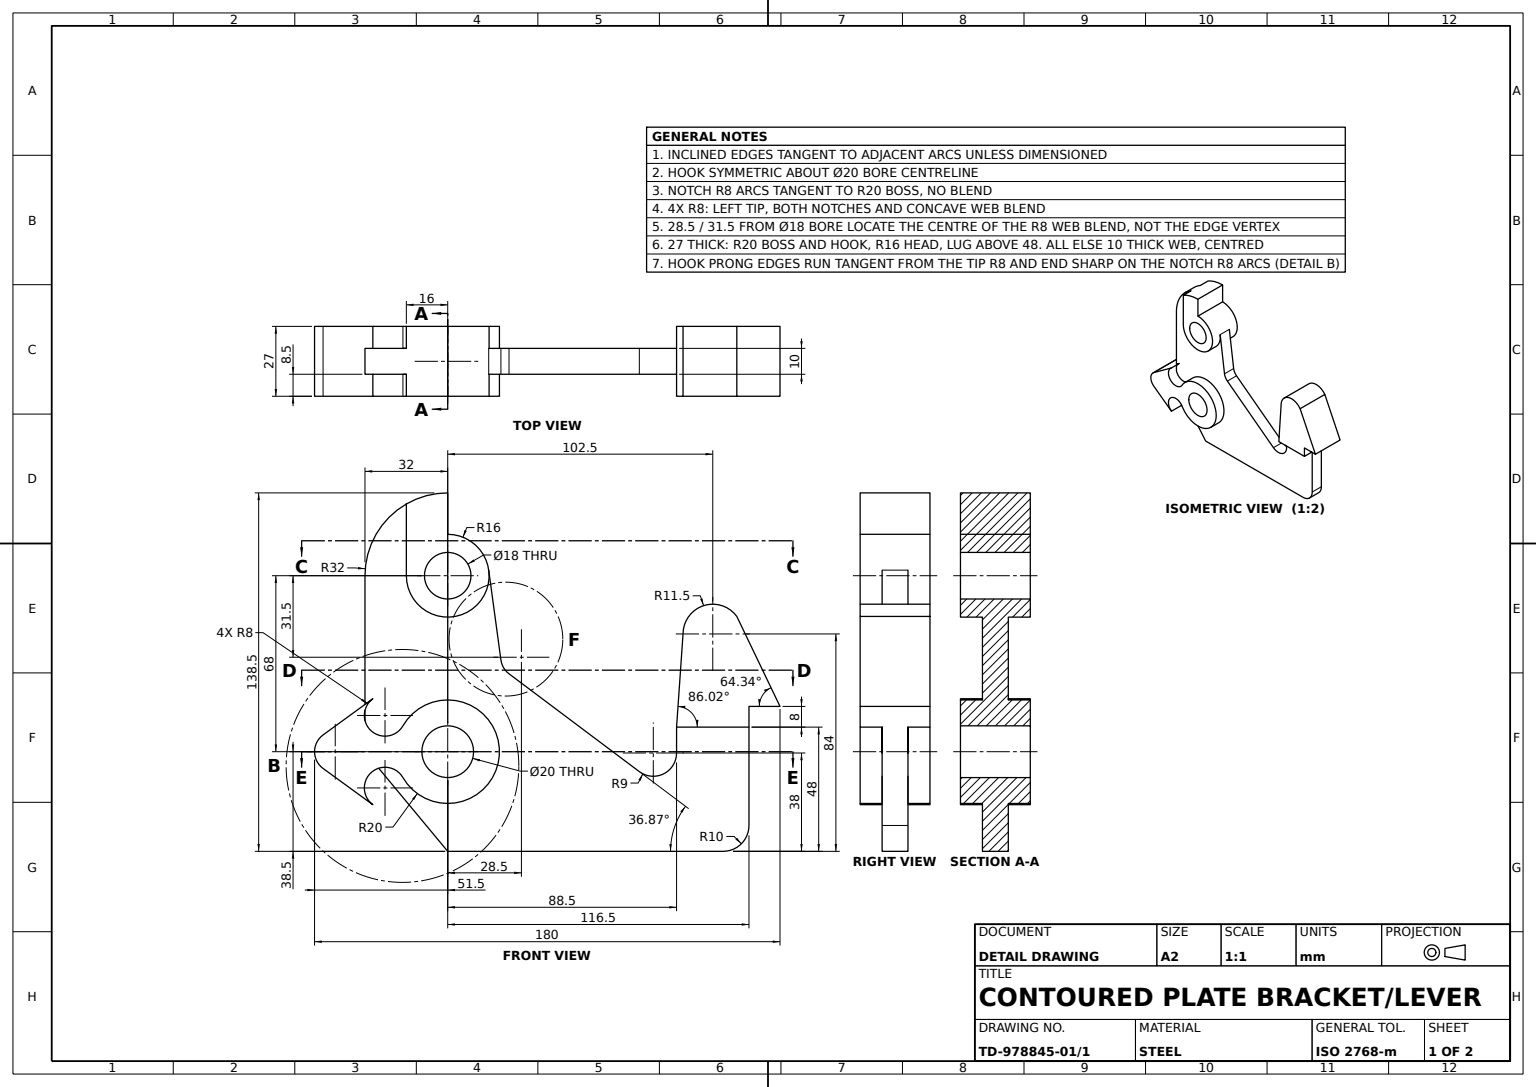
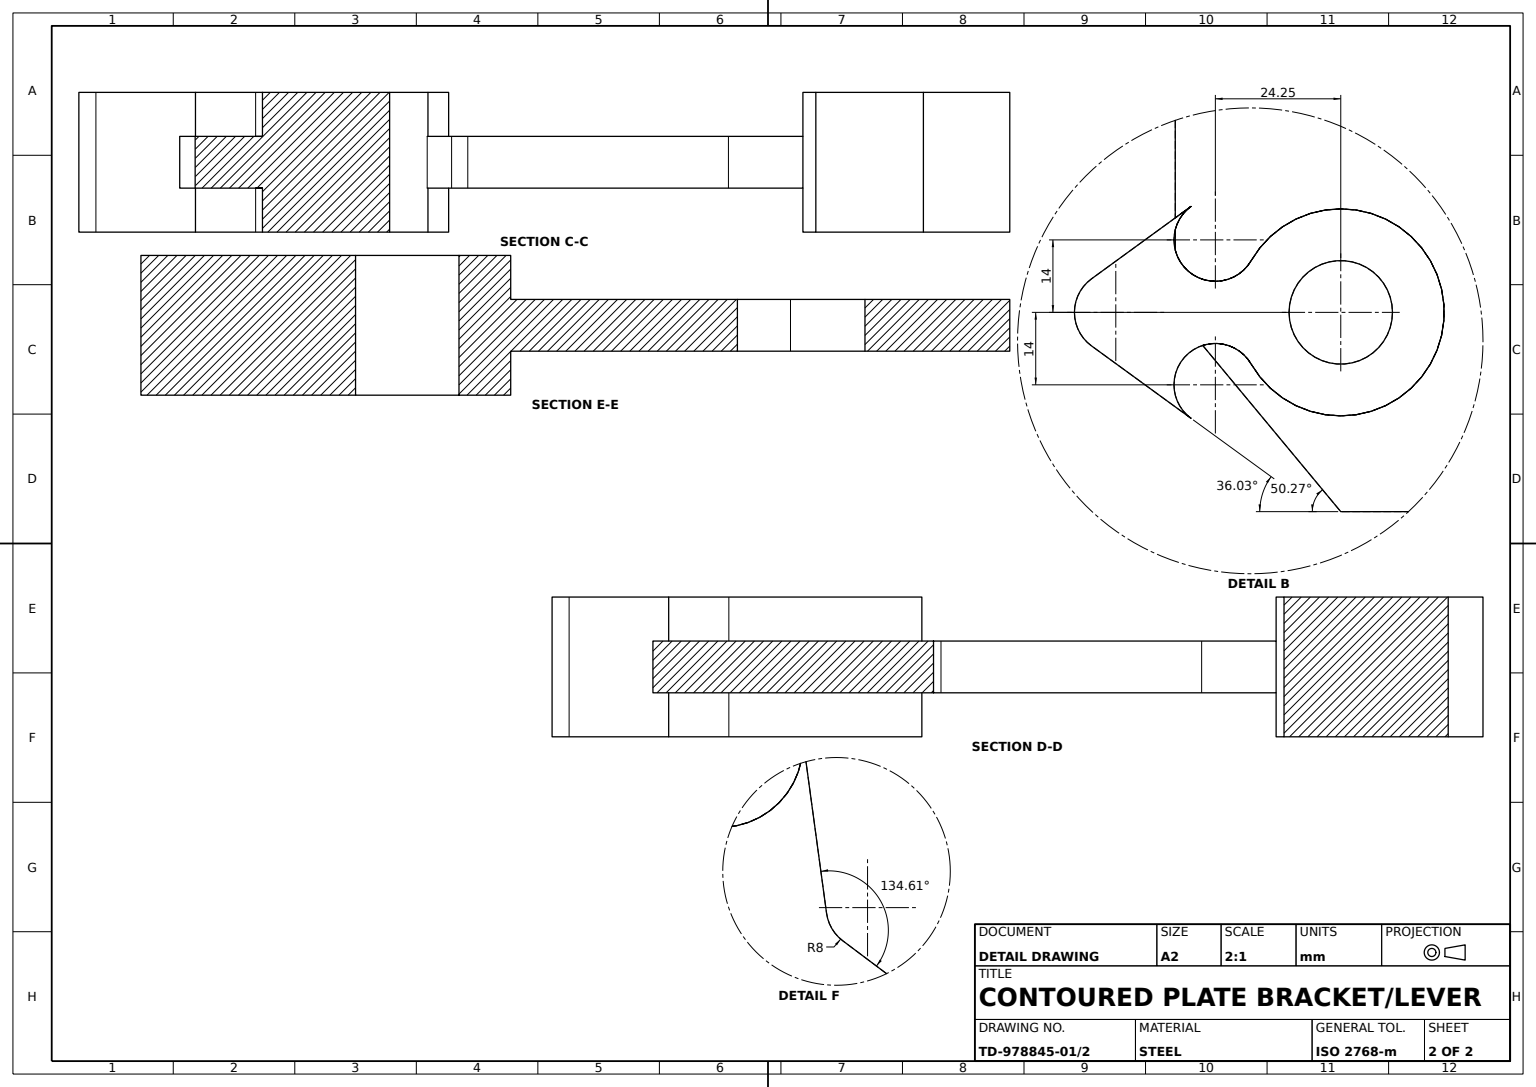
ISO-10303-21;
HEADER;
FILE_DESCRIPTION((''),'2;1');
FILE_NAME('','',(''),(''),'','','');
FILE_SCHEMA(('AUTOMOTIVE_DESIGN'));
ENDSEC;
DATA;
#1=APPLICATION_CONTEXT('');
#2=PRODUCT_CONTEXT('',#1,'mechanical');
#3=PRODUCT('','','',(#2));
#4=PRODUCT_DEFINITION_FORMATION('','',#3);
#5=PRODUCT_DEFINITION_CONTEXT('',#1,'design');
#6=PRODUCT_DEFINITION('','',#4,#5);
#7=PRODUCT_DEFINITION_SHAPE('','',#6);
#8=(LENGTH_UNIT()NAMED_UNIT(*)SI_UNIT(.MILLI.,.METRE.));
#9=(NAMED_UNIT(*)PLANE_ANGLE_UNIT()SI_UNIT($,.RADIAN.));
#10=(NAMED_UNIT(*)SI_UNIT($,.STERADIAN.)SOLID_ANGLE_UNIT());
#11=UNCERTAINTY_MEASURE_WITH_UNIT(LENGTH_MEASURE(1.E-05),#8,'distance_accuracy_value','');
#12=(GEOMETRIC_REPRESENTATION_CONTEXT(3)GLOBAL_UNCERTAINTY_ASSIGNED_CONTEXT((#11))GLOBAL_UNIT_ASSIGNED_CONTEXT((#8,#9,#10))REPRESENTATION_CONTEXT('',''));
#13=CARTESIAN_POINT('',(88.5,-58.5,-8.5));
#14=VERTEX_POINT('',#13);
#15=CARTESIAN_POINT('',(116.5,-58.5,-8.5));
#16=VERTEX_POINT('',#15);
#17=DIRECTION('',(1.,0.,0.));
#18=VECTOR('',#17,1000.);
#19=LINE('',#13,#18);
#20=EDGE_CURVE('',#14,#16,#19,.T.);
#21=ORIENTED_EDGE('',*,*,#20,.T.);
#22=CARTESIAN_POINT('',(116.5,-58.5,0.));
#23=VERTEX_POINT('',#22);
#24=CARTESIAN_POINT('',(116.5,-58.5,18.5));
#25=DIRECTION('',(0.,0.,-1.));
#26=VECTOR('',#25,1000.);
#27=LINE('',#24,#26);
#28=EDGE_CURVE('',#23,#16,#27,.T.);
#29=ORIENTED_EDGE('',*,*,#28,.F.);
#30=CARTESIAN_POINT('',(88.5,-58.5,0.));
#31=VERTEX_POINT('',#30);
#32=DIRECTION('',(-1.,0.,0.));
#33=VECTOR('',#32,1000.);
#34=LINE('',#22,#33);
#35=EDGE_CURVE('',#23,#31,#34,.T.);
#36=ORIENTED_EDGE('',*,*,#35,.T.);
#37=CARTESIAN_POINT('',(88.5,-58.5,18.5));
#38=LINE('',#37,#26);
#39=EDGE_CURVE('',#31,#14,#38,.T.);
#40=ORIENTED_EDGE('',*,*,#39,.T.);
#41=EDGE_LOOP('',(#21,#29,#36,#40));
#42=FACE_OUTER_BOUND('',#41,.T.);
#43=DIRECTION('',(0.,1.,0.));
#44=DIRECTION('',(0.,0.,1.));
#45=AXIS2_PLACEMENT_3D('',#37,#43,#44);
#46=PLANE('',#45);
#47=ADVANCED_FACE('',(#42),#46,.F.);
#48=CARTESIAN_POINT('',(128.5,-50.5,18.5));
#49=VERTEX_POINT('',#48);
#50=CARTESIAN_POINT('',(128.5,-50.5,-8.5));
#51=VERTEX_POINT('',#50);
#52=LINE('',#48,#26);
#53=EDGE_CURVE('',#49,#51,#52,.T.);
#54=ORIENTED_EDGE('',*,*,#53,.T.);
#55=CARTESIAN_POINT('',(111.797391,-15.731801,-8.5));
#56=VERTEX_POINT('',#55);
#57=DIRECTION('',(-0.433023369,0.901382695,0.));
#58=VECTOR('',#57,1000.);
#59=LINE('',#50,#58);
#60=EDGE_CURVE('',#51,#56,#59,.T.);
#61=ORIENTED_EDGE('',*,*,#60,.T.);
#62=CARTESIAN_POINT('',(111.797391,-15.731801,18.5));
#63=VERTEX_POINT('',#62);
#64=LINE('',#62,#26);
#65=EDGE_CURVE('',#63,#56,#64,.T.);
#66=ORIENTED_EDGE('',*,*,#65,.F.);
#67=LINE('',#48,#58);
#68=EDGE_CURVE('',#49,#63,#67,.T.);
#69=ORIENTED_EDGE('',*,*,#68,.F.);
#70=EDGE_LOOP('',(#54,#61,#66,#69));
#71=FACE_OUTER_BOUND('',#70,.T.);
#72=DIRECTION('',(-0.901382695,-0.433023369,0.));
#73=DIRECTION('',(0.433023369,-0.901382695,0.));
#74=AXIS2_PLACEMENT_3D('',#48,#72,#73);
#75=PLANE('',#74);
#76=ADVANCED_FACE('',(#71),#75,.F.);
#77=CARTESIAN_POINT('',(23.7,-37.9,10.));
#78=VERTEX_POINT('',#77);
#79=CARTESIAN_POINT('',(20.572823,-32.57697,10.));
#80=VERTEX_POINT('',#79);
#81=CARTESIAN_POINT('',(28.5,-31.5,10.));
#82=AXIS2_PLACEMENT_3D('',#81,#25,#17);
#83=CIRCLE('',#82,8.);
#84=EDGE_CURVE('',#78,#80,#83,.T.);
#85=ORIENTED_EDGE('',*,*,#84,.F.);
#86=CARTESIAN_POINT('',(23.7,-37.9,0.));
#87=VERTEX_POINT('',#86);
#88=LINE('',#77,#26);
#89=EDGE_CURVE('',#78,#87,#88,.T.);
#90=ORIENTED_EDGE('',*,*,#89,.T.);
#91=CARTESIAN_POINT('',(20.572823,-32.57697,0.));
#92=VERTEX_POINT('',#91);
#93=CARTESIAN_POINT('',(28.5,-31.5,0.));
#94=AXIS2_PLACEMENT_3D('',#93,#25,#17);
#95=CIRCLE('',#94,8.);
#96=EDGE_CURVE('',#87,#92,#95,.T.);
#97=ORIENTED_EDGE('',*,*,#96,.T.);
#98=LINE('',#79,#26);
#99=EDGE_CURVE('',#80,#92,#98,.T.);
#100=ORIENTED_EDGE('',*,*,#99,.F.);
#101=EDGE_LOOP('',(#85,#90,#97,#100));
#102=FACE_OUTER_BOUND('',#101,.T.);
#103=AXIS2_PLACEMENT_3D('',#81,#25,#32);
#104=CYLINDRICAL_SURFACE('',#103,8.);
#105=ADVANCED_FACE('',(#102),#104,.F.);
#106=CARTESIAN_POINT('',(-28.953879,-88.470039,18.5));
#107=VERTEX_POINT('',#106);
#108=CARTESIAN_POINT('',(-28.953879,-88.470039,-8.5));
#109=VERTEX_POINT('',#108);
#110=LINE('',#106,#26);
#111=EDGE_CURVE('',#107,#109,#110,.T.);
#112=ORIENTED_EDGE('',*,*,#111,.F.);
#113=CARTESIAN_POINT('',(-48.205168,-74.470039,18.5));
#114=VERTEX_POINT('',#113);
#115=DIRECTION('',(0.808754813,-0.588145945,0.));
#116=VECTOR('',#115,1000.);
#117=LINE('',#113,#116);
#118=EDGE_CURVE('',#114,#107,#117,.T.);
#119=ORIENTED_EDGE('',*,*,#118,.F.);
#120=CARTESIAN_POINT('',(-48.205168,-74.470039,-8.5));
#121=VERTEX_POINT('',#120);
#122=LINE('',#113,#26);
#123=EDGE_CURVE('',#114,#121,#122,.T.);
#124=ORIENTED_EDGE('',*,*,#123,.T.);
#125=LINE('',#120,#116);
#126=EDGE_CURVE('',#121,#109,#125,.T.);
#127=ORIENTED_EDGE('',*,*,#126,.T.);
#128=EDGE_LOOP('',(#112,#119,#124,#127));
#129=FACE_OUTER_BOUND('',#128,.T.);
#130=DIRECTION('',(0.588145945,0.808754813,0.));
#131=DIRECTION('',(-0.808754813,0.588145945,0.));
#132=AXIS2_PLACEMENT_3D('',#113,#130,#131);
#133=PLANE('',#132);
#134=ADVANCED_FACE('',(#129),#133,.F.);
#135=ORIENTED_EDGE('',*,*,#20,.F.);
#136=CARTESIAN_POINT('',(91.,-22.5,-8.5));
#137=VERTEX_POINT('',#136);
#138=DIRECTION('',(-0.069277599,-0.997597421,0.));
#139=VECTOR('',#138,1000.);
#140=LINE('',#136,#139);
#141=EDGE_CURVE('',#137,#14,#140,.T.);
#142=ORIENTED_EDGE('',*,*,#141,.F.);
#143=CARTESIAN_POINT('',(102.5,-22.5,-8.5));
#144=AXIS2_PLACEMENT_3D('',#143,#44,#17);
#145=CIRCLE('',#144,11.5);
#146=EDGE_CURVE('',#56,#137,#145,.T.);
#147=ORIENTED_EDGE('',*,*,#146,.F.);
#148=ORIENTED_EDGE('',*,*,#60,.F.);
#149=CARTESIAN_POINT('',(116.5,-50.5,-8.5));
#150=VERTEX_POINT('',#149);
#151=LINE('',#149,#18);
#152=EDGE_CURVE('',#150,#51,#151,.T.);
#153=ORIENTED_EDGE('',*,*,#152,.F.);
#154=VECTOR('',#43,1000.);
#155=LINE('',#15,#154);
#156=EDGE_CURVE('',#16,#150,#155,.T.);
#157=ORIENTED_EDGE('',*,*,#156,.F.);
#158=EDGE_LOOP('',(#135,#142,#147,#148,#153,#157));
#159=FACE_OUTER_BOUND('',#158,.T.);
#160=PLANE('',#144);
#161=ADVANCED_FACE('',(#159),#160,.F.);
#162=CARTESIAN_POINT('',(91.,-22.5,18.5));
#163=VERTEX_POINT('',#162);
#164=LINE('',#162,#26);
#165=EDGE_CURVE('',#163,#137,#164,.T.);
#166=ORIENTED_EDGE('',*,*,#165,.F.);
#167=CARTESIAN_POINT('',(102.5,-22.5,18.5));
#168=AXIS2_PLACEMENT_3D('',#167,#44,#17);
#169=CIRCLE('',#168,11.5);
#170=EDGE_CURVE('',#63,#163,#169,.T.);
#171=ORIENTED_EDGE('',*,*,#170,.F.);
#172=ORIENTED_EDGE('',*,*,#65,.T.);
#173=ORIENTED_EDGE('',*,*,#146,.T.);
#174=EDGE_LOOP('',(#166,#171,#172,#173));
#175=FACE_OUTER_BOUND('',#174,.T.);
#176=AXIS2_PLACEMENT_3D('',#167,#25,#32);
#177=CYLINDRICAL_SURFACE('',#176,11.5);
#178=ADVANCED_FACE('',(#175),#177,.T.);
#179=CARTESIAN_POINT('',(-32.248711,-82.,18.5));
#180=VERTEX_POINT('',#179);
#181=CARTESIAN_POINT('',(-24.248711,-82.,18.5));
#182=AXIS2_PLACEMENT_3D('',#181,#25,#17);
#183=CIRCLE('',#182,8.);
#184=EDGE_CURVE('',#107,#180,#183,.T.);
#185=ORIENTED_EDGE('',*,*,#184,.F.);
#186=ORIENTED_EDGE('',*,*,#111,.T.);
#187=CARTESIAN_POINT('',(-32.248711,-82.,-8.5));
#188=VERTEX_POINT('',#187);
#189=CARTESIAN_POINT('',(-24.248711,-82.,-8.5));
#190=AXIS2_PLACEMENT_3D('',#189,#25,#17);
#191=CIRCLE('',#190,8.);
#192=EDGE_CURVE('',#109,#188,#191,.T.);
#193=ORIENTED_EDGE('',*,*,#192,.T.);
#194=LINE('',#179,#26);
#195=EDGE_CURVE('',#180,#188,#194,.T.);
#196=ORIENTED_EDGE('',*,*,#195,.F.);
#197=EDGE_LOOP('',(#185,#186,#193,#196));
#198=FACE_OUTER_BOUND('',#197,.T.);
#199=AXIS2_PLACEMENT_3D('',#181,#25,#32);
#200=CYLINDRICAL_SURFACE('',#199,8.);
#201=ADVANCED_FACE('',(#198),#200,.F.);
#202=CARTESIAN_POINT('',(-17.320508,-58.,18.5));
#203=VERTEX_POINT('',#202);
#204=CARTESIAN_POINT('',(-17.320508,-58.,10.));
#205=VERTEX_POINT('',#204);
#206=LINE('',#202,#26);
#207=EDGE_CURVE('',#203,#205,#206,.T.);
#208=ORIENTED_EDGE('',*,*,#207,.F.);
#209=CARTESIAN_POINT('',(-17.320508,-78.,18.5));
#210=VERTEX_POINT('',#209);
#211=CARTESIAN_POINT('',(0.,-68.,18.5));
#212=AXIS2_PLACEMENT_3D('',#211,#44,#17);
#213=CIRCLE('',#212,20.);
#214=EDGE_CURVE('',#210,#203,#213,.T.);
#215=ORIENTED_EDGE('',*,*,#214,.F.);
#216=CARTESIAN_POINT('',(-17.320508,-78.,10.));
#217=VERTEX_POINT('',#216);
#218=LINE('',#209,#26);
#219=EDGE_CURVE('',#210,#217,#218,.T.);
#220=ORIENTED_EDGE('',*,*,#219,.T.);
#221=CARTESIAN_POINT('',(0.,-68.,10.));
#222=AXIS2_PLACEMENT_3D('',#221,#25,#17);
#223=CIRCLE('',#222,20.);
#224=EDGE_CURVE('',#205,#217,#223,.T.);
#225=ORIENTED_EDGE('',*,*,#224,.F.);
#226=EDGE_LOOP('',(#208,#215,#220,#225));
#227=FACE_OUTER_BOUND('',#226,.T.);
#228=AXIS2_PLACEMENT_3D('',#211,#25,#32);
#229=CYLINDRICAL_SURFACE('',#228,20.);
#230=ADVANCED_FACE('',(#227),#229,.T.);
#231=CARTESIAN_POINT('',(-17.320508,-58.,0.));
#232=VERTEX_POINT('',#231);
#233=CARTESIAN_POINT('',(-17.320508,-58.,-8.5));
#234=VERTEX_POINT('',#233);
#235=EDGE_CURVE('',#232,#234,#206,.T.);
#236=ORIENTED_EDGE('',*,*,#235,.F.);
#237=CARTESIAN_POINT('',(-17.320508,-78.,0.));
#238=VERTEX_POINT('',#237);
#239=CARTESIAN_POINT('',(0.,-68.,0.));
#240=AXIS2_PLACEMENT_3D('',#239,#25,#17);
#241=CIRCLE('',#240,20.);
#242=EDGE_CURVE('',#232,#238,#241,.T.);
#243=ORIENTED_EDGE('',*,*,#242,.T.);
#244=CARTESIAN_POINT('',(-17.320508,-78.,-8.5));
#245=VERTEX_POINT('',#244);
#246=EDGE_CURVE('',#238,#245,#218,.T.);
#247=ORIENTED_EDGE('',*,*,#246,.T.);
#248=CARTESIAN_POINT('',(0.,-68.,-8.5));
#249=AXIS2_PLACEMENT_3D('',#248,#44,#17);
#250=CIRCLE('',#249,20.);
#251=EDGE_CURVE('',#245,#234,#250,.T.);
#252=ORIENTED_EDGE('',*,*,#251,.T.);
#253=EDGE_LOOP('',(#236,#243,#247,#252));
#254=FACE_OUTER_BOUND('',#253,.T.);
#255=ADVANCED_FACE('',(#254),#229,.T.);
#256=VERTEX_POINT('',#37);
#257=VERTEX_POINT('',#24);
#258=LINE('',#37,#18);
#259=EDGE_CURVE('',#256,#257,#258,.T.);
#260=ORIENTED_EDGE('',*,*,#259,.T.);
#261=CARTESIAN_POINT('',(116.5,-50.5,18.5));
#262=VERTEX_POINT('',#261);
#263=LINE('',#24,#154);
#264=EDGE_CURVE('',#257,#262,#263,.T.);
#265=ORIENTED_EDGE('',*,*,#264,.T.);
#266=LINE('',#261,#18);
#267=EDGE_CURVE('',#262,#49,#266,.T.);
#268=ORIENTED_EDGE('',*,*,#267,.T.);
#269=ORIENTED_EDGE('',*,*,#68,.T.);
#270=ORIENTED_EDGE('',*,*,#170,.T.);
#271=LINE('',#162,#139);
#272=EDGE_CURVE('',#163,#256,#271,.T.);
#273=ORIENTED_EDGE('',*,*,#272,.T.);
#274=EDGE_LOOP('',(#260,#265,#268,#269,#270,#273));
#275=FACE_OUTER_BOUND('',#274,.T.);
#276=PLANE('',#168);
#277=ADVANCED_FACE('',(#275),#276,.T.);
#278=CARTESIAN_POINT('',(-32.,-49.745174,10.));
#279=VERTEX_POINT('',#278);
#280=CARTESIAN_POINT('',(-32.,-49.745174,0.));
#281=VERTEX_POINT('',#280);
#282=LINE('',#278,#26);
#283=EDGE_CURVE('',#279,#281,#282,.T.);
#284=ORIENTED_EDGE('',*,*,#283,.F.);
#285=CARTESIAN_POINT('',(-32.,0.,10.));
#286=VERTEX_POINT('',#285);
#287=DIRECTION('',(0.,-1.,0.));
#288=VECTOR('',#287,1000.);
#289=LINE('',#285,#288);
#290=EDGE_CURVE('',#286,#279,#289,.T.);
#291=ORIENTED_EDGE('',*,*,#290,.F.);
#292=CARTESIAN_POINT('',(-32.,0.,0.));
#293=VERTEX_POINT('',#292);
#294=LINE('',#285,#26);
#295=EDGE_CURVE('',#286,#293,#294,.T.);
#296=ORIENTED_EDGE('',*,*,#295,.T.);
#297=LINE('',#292,#288);
#298=EDGE_CURVE('',#293,#281,#297,.T.);
#299=ORIENTED_EDGE('',*,*,#298,.T.);
#300=EDGE_LOOP('',(#284,#291,#296,#299));
#301=FACE_OUTER_BOUND('',#300,.T.);
#302=AXIS2_PLACEMENT_3D('',#285,#17,#25);
#303=PLANE('',#302);
#304=ADVANCED_FACE('',(#301),#303,.F.);
#305=CARTESIAN_POINT('',(106.5,-106.5,10.));
#306=VERTEX_POINT('',#305);
#307=CARTESIAN_POINT('',(116.5,-96.5,10.));
#308=VERTEX_POINT('',#307);
#309=CARTESIAN_POINT('',(106.5,-96.5,10.));
#310=AXIS2_PLACEMENT_3D('',#309,#44,#17);
#311=CIRCLE('',#310,10.);
#312=EDGE_CURVE('',#306,#308,#311,.T.);
#313=ORIENTED_EDGE('',*,*,#312,.F.);
#314=CARTESIAN_POINT('',(106.5,-106.5,0.));
#315=VERTEX_POINT('',#314);
#316=VECTOR('',#44,1000.);
#317=LINE('',#305,#316);
#318=EDGE_CURVE('',#315,#306,#317,.T.);
#319=ORIENTED_EDGE('',*,*,#318,.F.);
#320=CARTESIAN_POINT('',(116.5,-96.5,0.));
#321=VERTEX_POINT('',#320);
#322=CARTESIAN_POINT('',(106.5,-96.5,0.));
#323=AXIS2_PLACEMENT_3D('',#322,#25,#17);
#324=CIRCLE('',#323,10.);
#325=EDGE_CURVE('',#321,#315,#324,.T.);
#326=ORIENTED_EDGE('',*,*,#325,.F.);
#327=LINE('',#307,#26);
#328=EDGE_CURVE('',#308,#321,#327,.T.);
#329=ORIENTED_EDGE('',*,*,#328,.F.);
#330=EDGE_LOOP('',(#313,#319,#326,#329));
#331=FACE_OUTER_BOUND('',#330,.T.);
#332=AXIS2_PLACEMENT_3D('',#309,#25,#32);
#333=CYLINDRICAL_SURFACE('',#332,10.);
#334=ADVANCED_FACE('',(#331),#333,.T.);
#335=CARTESIAN_POINT('',(-16.,27.712813,10.));
#336=VERTEX_POINT('',#335);
#337=CARTESIAN_POINT('',(0.,0.,10.));
#338=AXIS2_PLACEMENT_3D('',#337,#44,#17);
#339=CIRCLE('',#338,32.);
#340=EDGE_CURVE('',#336,#286,#339,.T.);
#341=ORIENTED_EDGE('',*,*,#340,.F.);
#342=CARTESIAN_POINT('',(-16.,27.712813,18.5));
#343=VERTEX_POINT('',#342);
#344=LINE('',#342,#26);
#345=EDGE_CURVE('',#343,#336,#344,.T.);
#346=ORIENTED_EDGE('',*,*,#345,.F.);
#347=CARTESIAN_POINT('',(0.,32.,18.5));
#348=VERTEX_POINT('',#347);
#349=CARTESIAN_POINT('',(0.,0.,18.5));
#350=AXIS2_PLACEMENT_3D('',#349,#44,#17);
#351=CIRCLE('',#350,32.);
#352=EDGE_CURVE('',#348,#343,#351,.T.);
#353=ORIENTED_EDGE('',*,*,#352,.F.);
#354=CARTESIAN_POINT('',(0.,32.,-8.5));
#355=VERTEX_POINT('',#354);
#356=CARTESIAN_POINT('',(0.,32.,10.));
#357=LINE('',#356,#26);
#358=EDGE_CURVE('',#348,#355,#357,.T.);
#359=ORIENTED_EDGE('',*,*,#358,.T.);
#360=CARTESIAN_POINT('',(-16.,27.712813,-8.5));
#361=VERTEX_POINT('',#360);
#362=CARTESIAN_POINT('',(0.,0.,-8.5));
#363=AXIS2_PLACEMENT_3D('',#362,#44,#17);
#364=CIRCLE('',#363,32.);
#365=EDGE_CURVE('',#355,#361,#364,.T.);
#366=ORIENTED_EDGE('',*,*,#365,.T.);
#367=CARTESIAN_POINT('',(-16.,27.712813,0.));
#368=VERTEX_POINT('',#367);
#369=EDGE_CURVE('',#368,#361,#344,.T.);
#370=ORIENTED_EDGE('',*,*,#369,.F.);
#371=CARTESIAN_POINT('',(0.,0.,0.));
#372=AXIS2_PLACEMENT_3D('',#371,#44,#17);
#373=CIRCLE('',#372,32.);
#374=EDGE_CURVE('',#368,#293,#373,.T.);
#375=ORIENTED_EDGE('',*,*,#374,.T.);
#376=ORIENTED_EDGE('',*,*,#295,.F.);
#377=EDGE_LOOP('',(#341,#346,#353,#359,#366,#370,#375,#376));
#378=FACE_OUTER_BOUND('',#377,.T.);
#379=AXIS2_PLACEMENT_3D('',#337,#25,#32);
#380=CYLINDRICAL_SURFACE('',#379,32.);
#381=ADVANCED_FACE('',(#378),#380,.T.);
#382=CARTESIAN_POINT('',(88.5,-58.5,10.));
#383=VERTEX_POINT('',#382);
#384=CARTESIAN_POINT('',(88.5,-68.5,10.));
#385=VERTEX_POINT('',#384);
#386=LINE('',#382,#288);
#387=EDGE_CURVE('',#383,#385,#386,.T.);
#388=ORIENTED_EDGE('',*,*,#387,.T.);
#389=CARTESIAN_POINT('',(74.1,-75.7,10.));
#390=VERTEX_POINT('',#389);
#391=CARTESIAN_POINT('',(79.5,-68.5,10.));
#392=AXIS2_PLACEMENT_3D('',#391,#25,#17);
#393=CIRCLE('',#392,9.);
#394=EDGE_CURVE('',#385,#390,#393,.T.);
#395=ORIENTED_EDGE('',*,*,#394,.T.);
#396=DIRECTION('',(-0.8,0.6,0.));
#397=VECTOR('',#396,1000.);
#398=LINE('',#77,#397);
#399=EDGE_CURVE('',#390,#78,#398,.T.);
#400=ORIENTED_EDGE('',*,*,#399,.T.);
#401=ORIENTED_EDGE('',*,*,#84,.T.);
#402=CARTESIAN_POINT('',(15.854354,2.153939,10.));
#403=VERTEX_POINT('',#402);
#404=DIRECTION('',(-0.134621216,0.990897133,0.));
#405=VECTOR('',#404,1000.);
#406=LINE('',#402,#405);
#407=EDGE_CURVE('',#80,#403,#406,.T.);
#408=ORIENTED_EDGE('',*,*,#407,.T.);
#409=CARTESIAN_POINT('',(-16.,0.,10.));
#410=VERTEX_POINT('',#409);
#411=AXIS2_PLACEMENT_3D('',#337,#25,#17);
#412=CIRCLE('',#411,16.);
#413=EDGE_CURVE('',#403,#410,#412,.T.);
#414=ORIENTED_EDGE('',*,*,#413,.T.);
#415=LINE('',#409,#154);
#416=EDGE_CURVE('',#410,#336,#415,.T.);
#417=ORIENTED_EDGE('',*,*,#416,.T.);
#418=ORIENTED_EDGE('',*,*,#340,.T.);
#419=ORIENTED_EDGE('',*,*,#290,.T.);
#420=CARTESIAN_POINT('',(-28.953879,-47.529961,10.));
#421=VERTEX_POINT('',#420);
#422=CARTESIAN_POINT('',(12.59278,-17.316232,10.));
#423=DIRECTION('',(0.808754813,0.588145945,0.));
#424=VECTOR('',#423,1000.);
#425=LINE('',#422,#424);
#426=EDGE_CURVE('',#279,#421,#425,.T.);
#427=ORIENTED_EDGE('',*,*,#426,.T.);
#428=CARTESIAN_POINT('',(-32.,-52.020727,10.));
#429=VERTEX_POINT('',#428);
#430=CARTESIAN_POINT('',(-24.248711,-54.,10.));
#431=AXIS2_PLACEMENT_3D('',#430,#44,#17);
#432=CIRCLE('',#431,8.);
#433=EDGE_CURVE('',#421,#429,#432,.T.);
#434=ORIENTED_EDGE('',*,*,#433,.T.);
#435=CARTESIAN_POINT('',(-32.,-55.979273,10.));
#436=VERTEX_POINT('',#435);
#437=EDGE_CURVE('',#429,#436,#289,.T.);
#438=ORIENTED_EDGE('',*,*,#437,.T.);
#439=EDGE_CURVE('',#436,#205,#432,.T.);
#440=ORIENTED_EDGE('',*,*,#439,.T.);
#441=ORIENTED_EDGE('',*,*,#224,.T.);
#442=CARTESIAN_POINT('',(-26.694593,-74.383067,10.));
#443=VERTEX_POINT('',#442);
#444=CARTESIAN_POINT('',(-24.248711,-82.,10.));
#445=AXIS2_PLACEMENT_3D('',#444,#44,#17);
#446=CIRCLE('',#445,8.);
#447=EDGE_CURVE('',#217,#443,#446,.T.);
#448=ORIENTED_EDGE('',*,*,#447,.T.);
#449=CARTESIAN_POINT('',(0.,-106.5,10.));
#450=VERTEX_POINT('',#449);
#451=CARTESIAN_POINT('',(-32.,-68.,10.));
#452=DIRECTION('',(0.639201497,-0.769039301,0.));
#453=VECTOR('',#452,1000.);
#454=LINE('',#451,#453);
#455=EDGE_CURVE('',#443,#450,#454,.T.);
#456=ORIENTED_EDGE('',*,*,#455,.T.);
#457=LINE('',#449,#18);
#458=EDGE_CURVE('',#450,#306,#457,.T.);
#459=ORIENTED_EDGE('',*,*,#458,.T.);
#460=ORIENTED_EDGE('',*,*,#312,.T.);
#461=CARTESIAN_POINT('',(116.5,-58.5,10.));
#462=VERTEX_POINT('',#461);
#463=CARTESIAN_POINT('',(116.5,-106.5,10.));
#464=LINE('',#463,#154);
#465=EDGE_CURVE('',#308,#462,#464,.T.);
#466=ORIENTED_EDGE('',*,*,#465,.T.);
#467=LINE('',#461,#33);
#468=EDGE_CURVE('',#462,#383,#467,.T.);
#469=ORIENTED_EDGE('',*,*,#468,.T.);
#470=EDGE_LOOP('',(#388,#395,#400,#401,#408,#414,#417,#418,#419,#427,#434,#438,#440,#441,#448,#456,#459,#460,#466,#469));
#471=FACE_OUTER_BOUND('',#470,.T.);
#472=PLANE('',#338);
#473=ADVANCED_FACE('',(#471),#472,.T.);
#474=CARTESIAN_POINT('',(-32.,-52.020727,0.));
#475=VERTEX_POINT('',#474);
#476=CARTESIAN_POINT('',(-32.,-52.020727,18.5));
#477=LINE('',#476,#316);
#478=EDGE_CURVE('',#475,#429,#477,.T.);
#479=ORIENTED_EDGE('',*,*,#478,.F.);
#480=CARTESIAN_POINT('',(-32.,-55.979273,0.));
#481=VERTEX_POINT('',#480);
#482=EDGE_CURVE('',#475,#481,#297,.T.);
#483=ORIENTED_EDGE('',*,*,#482,.T.);
#484=CARTESIAN_POINT('',(-32.,-55.979273,18.5));
#485=LINE('',#484,#26);
#486=EDGE_CURVE('',#436,#481,#485,.T.);
#487=ORIENTED_EDGE('',*,*,#486,.F.);
#488=ORIENTED_EDGE('',*,*,#437,.F.);
#489=EDGE_LOOP('',(#479,#483,#487,#488));
#490=FACE_OUTER_BOUND('',#489,.T.);
#491=ADVANCED_FACE('',(#490),#303,.F.);
#492=CARTESIAN_POINT('',(-32.248711,-54.,18.5));
#493=VERTEX_POINT('',#492);
#494=CARTESIAN_POINT('',(-24.248711,-54.,18.5));
#495=AXIS2_PLACEMENT_3D('',#494,#25,#17);
#496=CIRCLE('',#495,8.);
#497=EDGE_CURVE('',#203,#493,#496,.T.);
#498=ORIENTED_EDGE('',*,*,#497,.T.);
#499=CARTESIAN_POINT('',(-28.953879,-47.529961,18.5));
#500=VERTEX_POINT('',#499);
#501=EDGE_CURVE('',#493,#500,#496,.T.);
#502=ORIENTED_EDGE('',*,*,#501,.T.);
#503=CARTESIAN_POINT('',(-48.205168,-61.529961,18.5));
#504=VERTEX_POINT('',#503);
#505=DIRECTION('',(-0.808754813,-0.588145945,0.));
#506=VECTOR('',#505,1000.);
#507=LINE('',#503,#506);
#508=EDGE_CURVE('',#500,#504,#507,.T.);
#509=ORIENTED_EDGE('',*,*,#508,.T.);
#510=CARTESIAN_POINT('',(-51.5,-68.,18.5));
#511=VERTEX_POINT('',#510);
#512=CARTESIAN_POINT('',(-43.5,-68.,18.5));
#513=AXIS2_PLACEMENT_3D('',#512,#44,#17);
#514=CIRCLE('',#513,8.);
#515=EDGE_CURVE('',#504,#511,#514,.T.);
#516=ORIENTED_EDGE('',*,*,#515,.T.);
#517=EDGE_CURVE('',#511,#114,#514,.T.);
#518=ORIENTED_EDGE('',*,*,#517,.T.);
#519=ORIENTED_EDGE('',*,*,#118,.T.);
#520=ORIENTED_EDGE('',*,*,#184,.T.);
#521=EDGE_CURVE('',#180,#210,#183,.T.);
#522=ORIENTED_EDGE('',*,*,#521,.T.);
#523=ORIENTED_EDGE('',*,*,#214,.T.);
#524=EDGE_LOOP('',(#498,#502,#509,#516,#518,#519,#520,#522,#523));
#525=FACE_OUTER_BOUND('',#524,.T.);
#526=CARTESIAN_POINT('',(-10.,-68.,18.5));
#527=VERTEX_POINT('',#526);
#528=CARTESIAN_POINT('',(10.,-68.,18.5));
#529=VERTEX_POINT('',#528);
#530=CIRCLE('',#212,10.);
#531=EDGE_CURVE('',#527,#529,#530,.T.);
#532=ORIENTED_EDGE('',*,*,#531,.F.);
#533=EDGE_CURVE('',#529,#527,#530,.T.);
#534=ORIENTED_EDGE('',*,*,#533,.F.);
#535=EDGE_LOOP('',(#532,#534));
#536=FACE_BOUND('',#535,.T.);
#537=PLANE('',#513);
#538=ADVANCED_FACE('',(#525,#536),#537,.T.);
#539=ORIENTED_EDGE('',*,*,#99,.T.);
#540=CARTESIAN_POINT('',(15.854354,2.153939,0.));
#541=VERTEX_POINT('',#540);
#542=LINE('',#540,#405);
#543=EDGE_CURVE('',#92,#541,#542,.T.);
#544=ORIENTED_EDGE('',*,*,#543,.T.);
#545=LINE('',#402,#26);
#546=EDGE_CURVE('',#403,#541,#545,.T.);
#547=ORIENTED_EDGE('',*,*,#546,.F.);
#548=ORIENTED_EDGE('',*,*,#407,.F.);
#549=EDGE_LOOP('',(#539,#544,#547,#548));
#550=FACE_OUTER_BOUND('',#549,.T.);
#551=DIRECTION('',(-0.990897133,-0.134621216,0.));
#552=DIRECTION('',(0.134621216,-0.990897133,0.));
#553=AXIS2_PLACEMENT_3D('',#402,#551,#552);
#554=PLANE('',#553);
#555=ADVANCED_FACE('',(#550),#554,.F.);
#556=CARTESIAN_POINT('',(-51.5,-68.,-8.5));
#557=VERTEX_POINT('',#556);
#558=CARTESIAN_POINT('',(-43.5,-68.,-8.5));
#559=AXIS2_PLACEMENT_3D('',#558,#44,#17);
#560=CIRCLE('',#559,8.);
#561=EDGE_CURVE('',#557,#121,#560,.T.);
#562=ORIENTED_EDGE('',*,*,#561,.T.);
#563=ORIENTED_EDGE('',*,*,#123,.F.);
#564=ORIENTED_EDGE('',*,*,#517,.F.);
#565=LINE('',#510,#26);
#566=EDGE_CURVE('',#511,#557,#565,.T.);
#567=ORIENTED_EDGE('',*,*,#566,.T.);
#568=EDGE_LOOP('',(#562,#563,#564,#567));
#569=FACE_OUTER_BOUND('',#568,.T.);
#570=AXIS2_PLACEMENT_3D('',#512,#25,#32);
#571=CYLINDRICAL_SURFACE('',#570,8.);
#572=ADVANCED_FACE('',(#569),#571,.T.);
#573=ORIENTED_EDGE('',*,*,#39,.F.);
#574=LINE('',#382,#26);
#575=EDGE_CURVE('',#383,#31,#574,.T.);
#576=ORIENTED_EDGE('',*,*,#575,.F.);
#577=EDGE_CURVE('',#256,#383,#38,.T.);
#578=ORIENTED_EDGE('',*,*,#577,.F.);
#579=ORIENTED_EDGE('',*,*,#272,.F.);
#580=ORIENTED_EDGE('',*,*,#165,.T.);
#581=ORIENTED_EDGE('',*,*,#141,.T.);
#582=EDGE_LOOP('',(#573,#576,#578,#579,#580,#581));
#583=FACE_OUTER_BOUND('',#582,.T.);
#584=DIRECTION('',(0.997597421,-0.069277599,0.));
#585=DIRECTION('',(0.069277599,0.997597421,0.));
#586=AXIS2_PLACEMENT_3D('',#162,#584,#585);
#587=PLANE('',#586);
#588=ADVANCED_FACE('',(#583),#587,.F.);
#589=ORIENTED_EDGE('',*,*,#345,.T.);
#590=ORIENTED_EDGE('',*,*,#416,.F.);
#591=CARTESIAN_POINT('',(-16.,0.,18.5));
#592=VERTEX_POINT('',#591);
#593=LINE('',#591,#26);
#594=EDGE_CURVE('',#592,#410,#593,.T.);
#595=ORIENTED_EDGE('',*,*,#594,.F.);
#596=LINE('',#591,#288);
#597=EDGE_CURVE('',#343,#592,#596,.T.);
#598=ORIENTED_EDGE('',*,*,#597,.F.);
#599=EDGE_LOOP('',(#589,#590,#595,#598));
#600=FACE_OUTER_BOUND('',#599,.T.);
#601=AXIS2_PLACEMENT_3D('',#591,#17,#25);
#602=PLANE('',#601);
#603=ADVANCED_FACE('',(#600),#602,.F.);
#604=ORIENTED_EDGE('',*,*,#53,.F.);
#605=ORIENTED_EDGE('',*,*,#267,.F.);
#606=LINE('',#261,#26);
#607=EDGE_CURVE('',#262,#150,#606,.T.);
#608=ORIENTED_EDGE('',*,*,#607,.T.);
#609=ORIENTED_EDGE('',*,*,#152,.T.);
#610=EDGE_LOOP('',(#604,#605,#608,#609));
#611=FACE_OUTER_BOUND('',#610,.T.);
#612=AXIS2_PLACEMENT_3D('',#261,#43,#32);
#613=PLANE('',#612);
#614=ADVANCED_FACE('',(#611),#613,.F.);
#615=ORIENTED_EDGE('',*,*,#531,.T.);
#616=CARTESIAN_POINT('',(10.,-68.,-8.5));
#617=VERTEX_POINT('',#616);
#618=LINE('',#616,#316);
#619=EDGE_CURVE('',#617,#529,#618,.T.);
#620=ORIENTED_EDGE('',*,*,#619,.F.);
#621=CARTESIAN_POINT('',(-10.,-68.,-8.5));
#622=VERTEX_POINT('',#621);
#623=CIRCLE('',#249,10.);
#624=EDGE_CURVE('',#622,#617,#623,.T.);
#625=ORIENTED_EDGE('',*,*,#624,.F.);
#626=LINE('',#621,#316);
#627=EDGE_CURVE('',#622,#527,#626,.T.);
#628=ORIENTED_EDGE('',*,*,#627,.T.);
#629=EDGE_LOOP('',(#615,#620,#625,#628));
#630=FACE_OUTER_BOUND('',#629,.T.);
#631=CYLINDRICAL_SURFACE('',#249,10.);
#632=ADVANCED_FACE('',(#630),#631,.F.);
#633=CARTESIAN_POINT('',(116.5,-106.5,0.));
#634=LINE('',#633,#154);
#635=EDGE_CURVE('',#321,#23,#634,.T.);
#636=ORIENTED_EDGE('',*,*,#635,.T.);
#637=ORIENTED_EDGE('',*,*,#28,.T.);
#638=ORIENTED_EDGE('',*,*,#156,.T.);
#639=ORIENTED_EDGE('',*,*,#607,.F.);
#640=ORIENTED_EDGE('',*,*,#264,.F.);
#641=EDGE_CURVE('',#257,#462,#27,.T.);
#642=ORIENTED_EDGE('',*,*,#641,.T.);
#643=ORIENTED_EDGE('',*,*,#465,.F.);
#644=ORIENTED_EDGE('',*,*,#328,.T.);
#645=EDGE_LOOP('',(#636,#637,#638,#639,#640,#642,#643,#644));
#646=FACE_OUTER_BOUND('',#645,.T.);
#647=AXIS2_PLACEMENT_3D('',#463,#32,#44);
#648=PLANE('',#647);
#649=ADVANCED_FACE('',(#646),#648,.F.);
#650=ORIENTED_EDGE('',*,*,#521,.F.);
#651=ORIENTED_EDGE('',*,*,#195,.T.);
#652=EDGE_CURVE('',#188,#245,#191,.T.);
#653=ORIENTED_EDGE('',*,*,#652,.T.);
#654=ORIENTED_EDGE('',*,*,#246,.F.);
#655=CARTESIAN_POINT('',(-26.694593,-74.383067,0.));
#656=VERTEX_POINT('',#655);
#657=CARTESIAN_POINT('',(-24.248711,-82.,0.));
#658=AXIS2_PLACEMENT_3D('',#657,#44,#17);
#659=CIRCLE('',#658,8.);
#660=EDGE_CURVE('',#238,#656,#659,.T.);
#661=ORIENTED_EDGE('',*,*,#660,.T.);
#662=CARTESIAN_POINT('',(-26.694593,-74.383067,18.5));
#663=LINE('',#662,#316);
#664=EDGE_CURVE('',#656,#443,#663,.T.);
#665=ORIENTED_EDGE('',*,*,#664,.T.);
#666=ORIENTED_EDGE('',*,*,#447,.F.);
#667=ORIENTED_EDGE('',*,*,#219,.F.);
#668=EDGE_LOOP('',(#650,#651,#653,#654,#661,#665,#666,#667));
#669=FACE_OUTER_BOUND('',#668,.T.);
#670=ADVANCED_FACE('',(#669),#200,.F.);
#671=CARTESIAN_POINT('',(-28.953879,-47.529961,0.));
#672=VERTEX_POINT('',#671);
#673=CARTESIAN_POINT('',(-24.248711,-54.,0.));
#674=AXIS2_PLACEMENT_3D('',#673,#44,#17);
#675=CIRCLE('',#674,8.);
#676=EDGE_CURVE('',#672,#475,#675,.T.);
#677=ORIENTED_EDGE('',*,*,#676,.F.);
#678=CARTESIAN_POINT('',(12.59278,-17.316232,0.));
#679=LINE('',#678,#424);
#680=EDGE_CURVE('',#281,#672,#679,.T.);
#681=ORIENTED_EDGE('',*,*,#680,.F.);
#682=ORIENTED_EDGE('',*,*,#298,.F.);
#683=ORIENTED_EDGE('',*,*,#374,.F.);
#684=CARTESIAN_POINT('',(-16.,0.,0.));
#685=VERTEX_POINT('',#684);
#686=LINE('',#684,#154);
#687=EDGE_CURVE('',#685,#368,#686,.T.);
#688=ORIENTED_EDGE('',*,*,#687,.F.);
#689=AXIS2_PLACEMENT_3D('',#371,#25,#17);
#690=CIRCLE('',#689,16.);
#691=EDGE_CURVE('',#541,#685,#690,.T.);
#692=ORIENTED_EDGE('',*,*,#691,.F.);
#693=ORIENTED_EDGE('',*,*,#543,.F.);
#694=ORIENTED_EDGE('',*,*,#96,.F.);
#695=CARTESIAN_POINT('',(74.1,-75.7,0.));
#696=VERTEX_POINT('',#695);
#697=LINE('',#86,#397);
#698=EDGE_CURVE('',#696,#87,#697,.T.);
#699=ORIENTED_EDGE('',*,*,#698,.F.);
#700=CARTESIAN_POINT('',(88.5,-68.5,0.));
#701=VERTEX_POINT('',#700);
#702=CARTESIAN_POINT('',(79.5,-68.5,0.));
#703=AXIS2_PLACEMENT_3D('',#702,#25,#17);
#704=CIRCLE('',#703,9.);
#705=EDGE_CURVE('',#701,#696,#704,.T.);
#706=ORIENTED_EDGE('',*,*,#705,.F.);
#707=LINE('',#30,#288);
#708=EDGE_CURVE('',#31,#701,#707,.T.);
#709=ORIENTED_EDGE('',*,*,#708,.F.);
#710=ORIENTED_EDGE('',*,*,#35,.F.);
#711=ORIENTED_EDGE('',*,*,#635,.F.);
#712=ORIENTED_EDGE('',*,*,#325,.T.);
#713=CARTESIAN_POINT('',(0.,-106.5,0.));
#714=VERTEX_POINT('',#713);
#715=LINE('',#713,#18);
#716=EDGE_CURVE('',#714,#315,#715,.T.);
#717=ORIENTED_EDGE('',*,*,#716,.F.);
#718=CARTESIAN_POINT('',(-32.,-68.,0.));
#719=LINE('',#718,#453);
#720=EDGE_CURVE('',#656,#714,#719,.T.);
#721=ORIENTED_EDGE('',*,*,#720,.F.);
#722=ORIENTED_EDGE('',*,*,#660,.F.);
#723=ORIENTED_EDGE('',*,*,#242,.F.);
#724=EDGE_CURVE('',#481,#232,#675,.T.);
#725=ORIENTED_EDGE('',*,*,#724,.F.);
#726=ORIENTED_EDGE('',*,*,#482,.F.);
#727=EDGE_LOOP('',(#677,#681,#682,#683,#688,#692,#693,#694,#699,#706,#709,#710,#711,#712,#717,#721,#722,#723,#725,#726));
#728=FACE_OUTER_BOUND('',#727,.T.);
#729=PLANE('',#372);
#730=ADVANCED_FACE('',(#728),#729,.F.);
#731=ORIENTED_EDGE('',*,*,#627,.F.);
#732=EDGE_CURVE('',#617,#622,#623,.T.);
#733=ORIENTED_EDGE('',*,*,#732,.F.);
#734=ORIENTED_EDGE('',*,*,#619,.T.);
#735=ORIENTED_EDGE('',*,*,#533,.T.);
#736=EDGE_LOOP('',(#731,#733,#734,#735));
#737=FACE_OUTER_BOUND('',#736,.T.);
#738=ADVANCED_FACE('',(#737),#631,.F.);
#739=CARTESIAN_POINT('',(9.,0.,18.5));
#740=VERTEX_POINT('',#739);
#741=CARTESIAN_POINT('',(-9.,0.,18.5));
#742=VERTEX_POINT('',#741);
#743=CIRCLE('',#350,9.);
#744=EDGE_CURVE('',#740,#742,#743,.T.);
#745=ORIENTED_EDGE('',*,*,#744,.T.);
#746=CARTESIAN_POINT('',(-9.,0.,-8.5));
#747=VERTEX_POINT('',#746);
#748=LINE('',#746,#316);
#749=EDGE_CURVE('',#747,#742,#748,.T.);
#750=ORIENTED_EDGE('',*,*,#749,.F.);
#751=CARTESIAN_POINT('',(9.,0.,-8.5));
#752=VERTEX_POINT('',#751);
#753=CIRCLE('',#363,9.);
#754=EDGE_CURVE('',#752,#747,#753,.T.);
#755=ORIENTED_EDGE('',*,*,#754,.F.);
#756=LINE('',#751,#316);
#757=EDGE_CURVE('',#752,#740,#756,.T.);
#758=ORIENTED_EDGE('',*,*,#757,.T.);
#759=EDGE_LOOP('',(#745,#750,#755,#758));
#760=FACE_OUTER_BOUND('',#759,.T.);
#761=CYLINDRICAL_SURFACE('',#363,9.);
#762=ADVANCED_FACE('',(#760),#761,.F.);
#763=ORIENTED_EDGE('',*,*,#455,.F.);
#764=ORIENTED_EDGE('',*,*,#664,.F.);
#765=ORIENTED_EDGE('',*,*,#720,.T.);
#766=LINE('',#449,#26);
#767=EDGE_CURVE('',#450,#714,#766,.T.);
#768=ORIENTED_EDGE('',*,*,#767,.F.);
#769=EDGE_LOOP('',(#763,#764,#765,#768));
#770=FACE_OUTER_BOUND('',#769,.T.);
#771=DIRECTION('',(0.769039301,0.639201497,0.));
#772=DIRECTION('',(-0.639201497,0.769039301,0.));
#773=AXIS2_PLACEMENT_3D('',#451,#771,#772);
#774=PLANE('',#773);
#775=ADVANCED_FACE('',(#770),#774,.F.);
#776=ORIENTED_EDGE('',*,*,#624,.T.);
#777=ORIENTED_EDGE('',*,*,#732,.T.);
#778=EDGE_LOOP('',(#776,#777));
#779=FACE_BOUND('',#778,.T.);
#780=ORIENTED_EDGE('',*,*,#652,.F.);
#781=ORIENTED_EDGE('',*,*,#192,.F.);
#782=ORIENTED_EDGE('',*,*,#126,.F.);
#783=ORIENTED_EDGE('',*,*,#561,.F.);
#784=CARTESIAN_POINT('',(-48.205168,-61.529961,-8.5));
#785=VERTEX_POINT('',#784);
#786=EDGE_CURVE('',#785,#557,#560,.T.);
#787=ORIENTED_EDGE('',*,*,#786,.F.);
#788=CARTESIAN_POINT('',(-28.953879,-47.529961,-8.5));
#789=VERTEX_POINT('',#788);
#790=LINE('',#784,#506);
#791=EDGE_CURVE('',#789,#785,#790,.T.);
#792=ORIENTED_EDGE('',*,*,#791,.F.);
#793=CARTESIAN_POINT('',(-32.248711,-54.,-8.5));
#794=VERTEX_POINT('',#793);
#795=CARTESIAN_POINT('',(-24.248711,-54.,-8.5));
#796=AXIS2_PLACEMENT_3D('',#795,#25,#17);
#797=CIRCLE('',#796,8.);
#798=EDGE_CURVE('',#794,#789,#797,.T.);
#799=ORIENTED_EDGE('',*,*,#798,.F.);
#800=EDGE_CURVE('',#234,#794,#797,.T.);
#801=ORIENTED_EDGE('',*,*,#800,.F.);
#802=ORIENTED_EDGE('',*,*,#251,.F.);
#803=EDGE_LOOP('',(#780,#781,#782,#783,#787,#792,#799,#801,#802));
#804=FACE_OUTER_BOUND('',#803,.T.);
#805=PLANE('',#559);
#806=ADVANCED_FACE('',(#779,#804),#805,.F.);
#807=LINE('',#384,#26);
#808=EDGE_CURVE('',#385,#701,#807,.T.);
#809=ORIENTED_EDGE('',*,*,#808,.F.);
#810=ORIENTED_EDGE('',*,*,#387,.F.);
#811=ORIENTED_EDGE('',*,*,#575,.T.);
#812=ORIENTED_EDGE('',*,*,#708,.T.);
#813=EDGE_LOOP('',(#809,#810,#811,#812));
#814=FACE_OUTER_BOUND('',#813,.T.);
#815=AXIS2_PLACEMENT_3D('',#382,#17,#43);
#816=PLANE('',#815);
#817=ADVANCED_FACE('',(#814),#816,.F.);
#818=ORIENTED_EDGE('',*,*,#698,.T.);
#819=ORIENTED_EDGE('',*,*,#89,.F.);
#820=ORIENTED_EDGE('',*,*,#399,.F.);
#821=LINE('',#389,#26);
#822=EDGE_CURVE('',#390,#696,#821,.T.);
#823=ORIENTED_EDGE('',*,*,#822,.T.);
#824=EDGE_LOOP('',(#818,#819,#820,#823));
#825=FACE_OUTER_BOUND('',#824,.T.);
#826=DIRECTION('',(-0.6,-0.8,0.));
#827=DIRECTION('',(0.8,-0.6,0.));
#828=AXIS2_PLACEMENT_3D('',#77,#826,#827);
#829=PLANE('',#828);
#830=ADVANCED_FACE('',(#825),#829,.F.);
#831=ORIENTED_EDGE('',*,*,#786,.T.);
#832=ORIENTED_EDGE('',*,*,#566,.F.);
#833=ORIENTED_EDGE('',*,*,#515,.F.);
#834=LINE('',#503,#26);
#835=EDGE_CURVE('',#504,#785,#834,.T.);
#836=ORIENTED_EDGE('',*,*,#835,.T.);
#837=EDGE_LOOP('',(#831,#832,#833,#836));
#838=FACE_OUTER_BOUND('',#837,.T.);
#839=ADVANCED_FACE('',(#838),#571,.T.);
#840=ORIENTED_EDGE('',*,*,#680,.T.);
#841=LINE('',#499,#26);
#842=EDGE_CURVE('',#672,#789,#841,.T.);
#843=ORIENTED_EDGE('',*,*,#842,.T.);
#844=ORIENTED_EDGE('',*,*,#791,.T.);
#845=ORIENTED_EDGE('',*,*,#835,.F.);
#846=ORIENTED_EDGE('',*,*,#508,.F.);
#847=EDGE_CURVE('',#500,#421,#841,.T.);
#848=ORIENTED_EDGE('',*,*,#847,.T.);
#849=ORIENTED_EDGE('',*,*,#426,.F.);
#850=ORIENTED_EDGE('',*,*,#283,.T.);
#851=EDGE_LOOP('',(#840,#843,#844,#845,#846,#848,#849,#850));
#852=FACE_OUTER_BOUND('',#851,.T.);
#853=DIRECTION('',(0.588145945,-0.808754813,0.));
#854=AXIS2_PLACEMENT_3D('',#503,#853,#423);
#855=PLANE('',#854);
#856=ADVANCED_FACE('',(#852),#855,.F.);
#857=CARTESIAN_POINT('',(0.,16.,-8.5));
#858=VERTEX_POINT('',#857);
#859=LINE('',#857,#154);
#860=EDGE_CURVE('',#858,#355,#859,.T.);
#861=ORIENTED_EDGE('',*,*,#860,.T.);
#862=ORIENTED_EDGE('',*,*,#358,.F.);
#863=CARTESIAN_POINT('',(0.,16.,18.5));
#864=VERTEX_POINT('',#863);
#865=LINE('',#863,#154);
#866=EDGE_CURVE('',#864,#348,#865,.T.);
#867=ORIENTED_EDGE('',*,*,#866,.F.);
#868=CARTESIAN_POINT('',(0.,16.,10.));
#869=LINE('',#868,#26);
#870=EDGE_CURVE('',#864,#858,#869,.T.);
#871=ORIENTED_EDGE('',*,*,#870,.T.);
#872=EDGE_LOOP('',(#861,#862,#867,#871));
#873=FACE_OUTER_BOUND('',#872,.T.);
#874=AXIS2_PLACEMENT_3D('',#868,#32,#44);
#875=PLANE('',#874);
#876=ADVANCED_FACE('',(#873),#875,.F.);
#877=ORIENTED_EDGE('',*,*,#641,.F.);
#878=ORIENTED_EDGE('',*,*,#259,.F.);
#879=ORIENTED_EDGE('',*,*,#577,.T.);
#880=ORIENTED_EDGE('',*,*,#468,.F.);
#881=EDGE_LOOP('',(#877,#878,#879,#880));
#882=FACE_OUTER_BOUND('',#881,.T.);
#883=ADVANCED_FACE('',(#882),#46,.F.);
#884=CARTESIAN_POINT('',(-16.,0.,-8.5));
#885=VERTEX_POINT('',#884);
#886=EDGE_CURVE('',#685,#885,#593,.T.);
#887=ORIENTED_EDGE('',*,*,#886,.T.);
#888=CIRCLE('',#363,16.);
#889=EDGE_CURVE('',#885,#858,#888,.T.);
#890=ORIENTED_EDGE('',*,*,#889,.T.);
#891=ORIENTED_EDGE('',*,*,#870,.F.);
#892=CIRCLE('',#350,16.);
#893=EDGE_CURVE('',#592,#864,#892,.T.);
#894=ORIENTED_EDGE('',*,*,#893,.F.);
#895=ORIENTED_EDGE('',*,*,#594,.T.);
#896=ORIENTED_EDGE('',*,*,#413,.F.);
#897=ORIENTED_EDGE('',*,*,#546,.T.);
#898=ORIENTED_EDGE('',*,*,#691,.T.);
#899=EDGE_LOOP('',(#887,#890,#891,#894,#895,#896,#897,#898));
#900=FACE_OUTER_BOUND('',#899,.T.);
#901=CYLINDRICAL_SURFACE('',#379,16.);
#902=ADVANCED_FACE('',(#900),#901,.T.);
#903=LINE('',#884,#288);
#904=EDGE_CURVE('',#361,#885,#903,.T.);
#905=ORIENTED_EDGE('',*,*,#904,.T.);
#906=ORIENTED_EDGE('',*,*,#886,.F.);
#907=ORIENTED_EDGE('',*,*,#687,.T.);
#908=ORIENTED_EDGE('',*,*,#369,.T.);
#909=EDGE_LOOP('',(#905,#906,#907,#908));
#910=FACE_OUTER_BOUND('',#909,.T.);
#911=ADVANCED_FACE('',(#910),#602,.F.);
#912=ORIENTED_EDGE('',*,*,#478,.T.);
#913=ORIENTED_EDGE('',*,*,#433,.F.);
#914=ORIENTED_EDGE('',*,*,#847,.F.);
#915=ORIENTED_EDGE('',*,*,#501,.F.);
#916=LINE('',#492,#26);
#917=EDGE_CURVE('',#493,#794,#916,.T.);
#918=ORIENTED_EDGE('',*,*,#917,.T.);
#919=ORIENTED_EDGE('',*,*,#798,.T.);
#920=ORIENTED_EDGE('',*,*,#842,.F.);
#921=ORIENTED_EDGE('',*,*,#676,.T.);
#922=EDGE_LOOP('',(#912,#913,#914,#915,#918,#919,#920,#921));
#923=FACE_OUTER_BOUND('',#922,.T.);
#924=AXIS2_PLACEMENT_3D('',#494,#25,#32);
#925=CYLINDRICAL_SURFACE('',#924,8.);
#926=ADVANCED_FACE('',(#923),#925,.F.);
#927=ORIENTED_EDGE('',*,*,#749,.T.);
#928=EDGE_CURVE('',#742,#740,#743,.T.);
#929=ORIENTED_EDGE('',*,*,#928,.T.);
#930=ORIENTED_EDGE('',*,*,#757,.F.);
#931=EDGE_CURVE('',#747,#752,#753,.T.);
#932=ORIENTED_EDGE('',*,*,#931,.F.);
#933=EDGE_LOOP('',(#927,#929,#930,#932));
#934=FACE_OUTER_BOUND('',#933,.T.);
#935=ADVANCED_FACE('',(#934),#761,.F.);
#936=ORIENTED_EDGE('',*,*,#822,.F.);
#937=ORIENTED_EDGE('',*,*,#394,.F.);
#938=ORIENTED_EDGE('',*,*,#808,.T.);
#939=ORIENTED_EDGE('',*,*,#705,.T.);
#940=EDGE_LOOP('',(#936,#937,#938,#939));
#941=FACE_OUTER_BOUND('',#940,.T.);
#942=AXIS2_PLACEMENT_3D('',#391,#25,#32);
#943=CYLINDRICAL_SURFACE('',#942,9.);
#944=ADVANCED_FACE('',(#941),#943,.F.);
#945=ORIENTED_EDGE('',*,*,#866,.T.);
#946=ORIENTED_EDGE('',*,*,#352,.T.);
#947=ORIENTED_EDGE('',*,*,#597,.T.);
#948=ORIENTED_EDGE('',*,*,#893,.T.);
#949=EDGE_LOOP('',(#945,#946,#947,#948));
#950=FACE_OUTER_BOUND('',#949,.T.);
#951=ORIENTED_EDGE('',*,*,#744,.F.);
#952=ORIENTED_EDGE('',*,*,#928,.F.);
#953=EDGE_LOOP('',(#951,#952));
#954=FACE_BOUND('',#953,.T.);
#955=PLANE('',#350);
#956=ADVANCED_FACE('',(#950,#954),#955,.T.);
#957=ORIENTED_EDGE('',*,*,#889,.F.);
#958=ORIENTED_EDGE('',*,*,#904,.F.);
#959=ORIENTED_EDGE('',*,*,#365,.F.);
#960=ORIENTED_EDGE('',*,*,#860,.F.);
#961=EDGE_LOOP('',(#957,#958,#959,#960));
#962=FACE_OUTER_BOUND('',#961,.T.);
#963=ORIENTED_EDGE('',*,*,#931,.T.);
#964=ORIENTED_EDGE('',*,*,#754,.T.);
#965=EDGE_LOOP('',(#963,#964));
#966=FACE_BOUND('',#965,.T.);
#967=PLANE('',#363);
#968=ADVANCED_FACE('',(#962,#966),#967,.F.);
#969=ORIENTED_EDGE('',*,*,#318,.T.);
#970=ORIENTED_EDGE('',*,*,#458,.F.);
#971=ORIENTED_EDGE('',*,*,#767,.T.);
#972=ORIENTED_EDGE('',*,*,#716,.T.);
#973=EDGE_LOOP('',(#969,#970,#971,#972));
#974=FACE_OUTER_BOUND('',#973,.T.);
#975=AXIS2_PLACEMENT_3D('',#449,#43,#44);
#976=PLANE('',#975);
#977=ADVANCED_FACE('',(#974),#976,.F.);
#978=ORIENTED_EDGE('',*,*,#917,.F.);
#979=ORIENTED_EDGE('',*,*,#497,.F.);
#980=ORIENTED_EDGE('',*,*,#207,.T.);
#981=ORIENTED_EDGE('',*,*,#439,.F.);
#982=ORIENTED_EDGE('',*,*,#486,.T.);
#983=ORIENTED_EDGE('',*,*,#724,.T.);
#984=ORIENTED_EDGE('',*,*,#235,.T.);
#985=ORIENTED_EDGE('',*,*,#800,.T.);
#986=EDGE_LOOP('',(#978,#979,#980,#981,#982,#983,#984,#985));
#987=FACE_OUTER_BOUND('',#986,.T.);
#988=ADVANCED_FACE('',(#987),#925,.F.);
#989=CLOSED_SHELL('',(#47,#76,#105,#134,#161,#178,#201,#230,#255,#277,#304,#334,#381,#473,#491,#538,#555,#572,#588,#603,#614,#632,#649,#670,#730,#738,#762,#775,#806,#817,#830,#839,#856,#876,#883,#902,#911,#926,#935,#944,#956,#968,#977,#988));
#990=MANIFOLD_SOLID_BREP('',#989);
#991=ADVANCED_BREP_SHAPE_REPRESENTATION('',(#990),#12);
#992=SHAPE_DEFINITION_REPRESENTATION(#7,#991);
ENDSEC;
END-ISO-10303-21;
